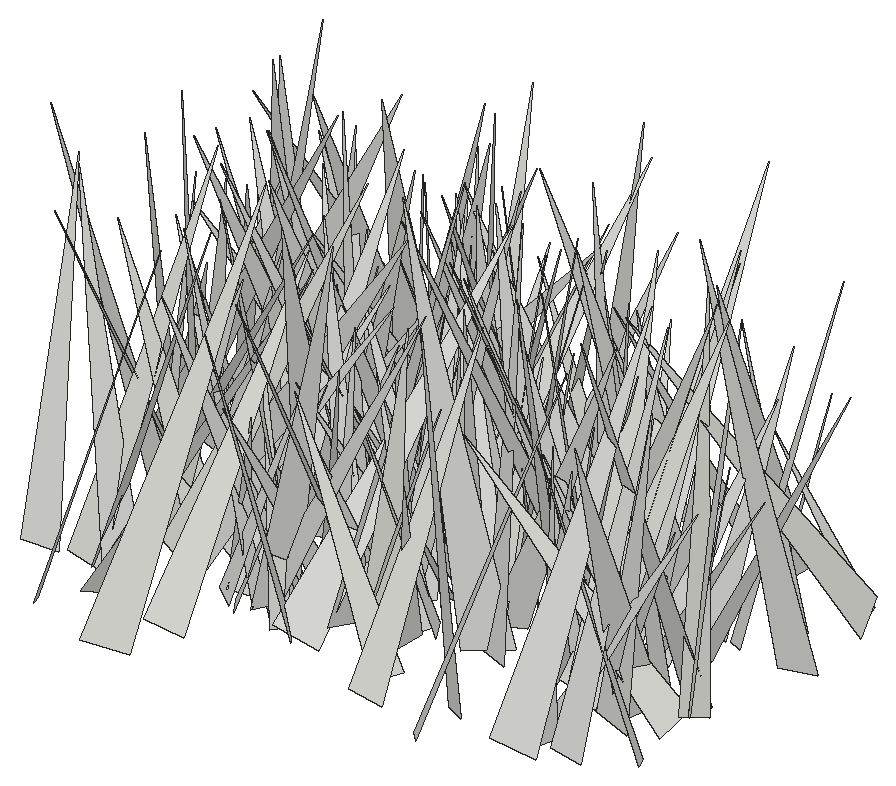
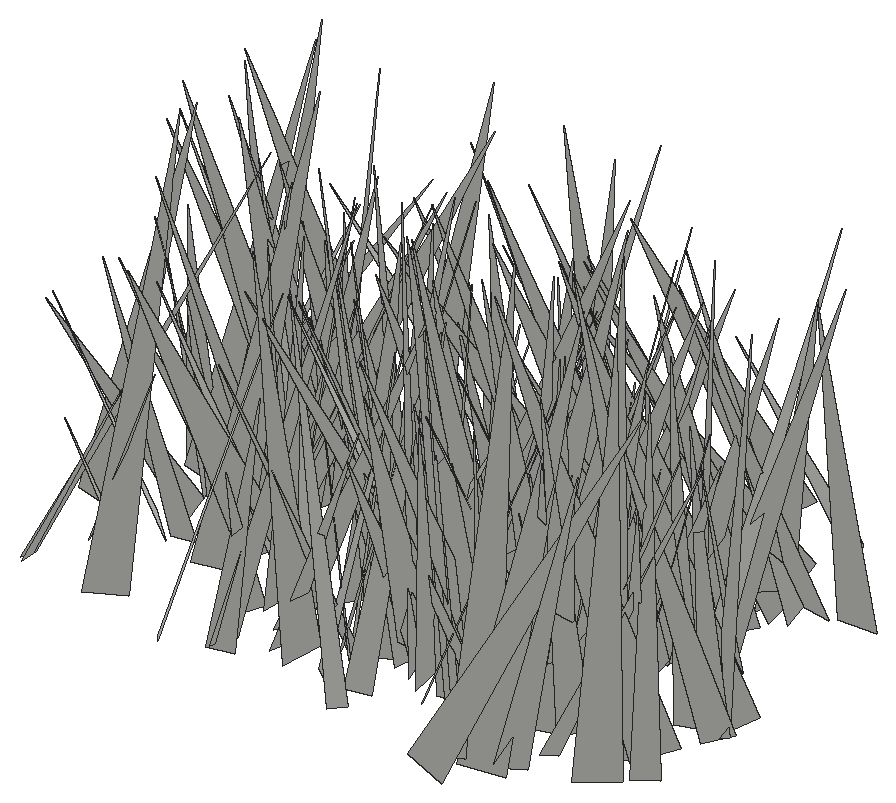
# SketchUp Ruby script. Lengths in inches.
U = 1.inch
M = Sketchup.active_model
def pt(a) = Geom::Point3d.new(a.map { |v| v * U })
def face(e, loops, mat)
  f = e.add_face(loops[0].map { |a| pt(a) })
  loops[1..].each { |l| e.add_face(l.map { |a| pt(a) }).erase! }
  f.material = f.back_material = mat if mat
  f
end
# faces: each face lists its corners as indices into pts; further lists are holes
def faces(e, pts, list, mat = nil) = list.each { |f| face(e, (f[0].is_a?(Array) ? f : [f]).map { |l| l.map { |i| pts[i] } }, mat) }
# xy, xz, yz: faces in a plane at the given z, y or x. An outline is a flat list of corners, or four numbers for a rectangle; further outlines are holes
def ring(l) = l.size == 4 ? [[l[0], l[1]], [l[2], l[1]], [l[2], l[3]], [l[0], l[3]]] : l.each_slice(2).to_a
def flat(e, list, mat, &to3) = list.each { |f| face(e, (f[0].is_a?(Array) ? f : [f]).map { |l| ring(l).map { |u, v| to3.(u, v) } }, mat) }
def xy(e, z, list, mat = nil) = flat(e, list, mat) { |x, y| [x, y, z] }
def xz(e, y, list, mat = nil) = flat(e, list, mat) { |x, z| [x, y, z] }
def yz(e, x, list, mat = nil) = flat(e, list, mat) { |y, z| [x, y, z] }
def lines(e, pts, list) = list.each { |a, b| e.add_line(pt(pts[a]), pt(pts[b])) }
# prism: a flat outline (further loops are holes) pulled along v
def prism(e, loops, v, mat = nil)
  f = face(e, loops, mat); d = Geom::Vector3d.new(v.map { |x| x * U })
  f.pushpull(f.normal.samedirection?(d) ? d.length : -d.length)
end
def box(e, o, s, mat = nil) = prism(e, [[o, [o[0] + s[0], o[1], o[2]], [o[0] + s[0], o[1] + s[1], o[2]], [o[0], o[1] + s[1], o[2]]]], [0, 0, s[2]], mat)
def at(x, y, z, deg = 0) = Geom::Transformation.translation(pt([x, y, z])) * Geom::Transformation.rotation(ORIGIN, Z_AXIS, deg.degrees)
def axes(o, x, y, z) = Geom::Transformation.new([*x, 0, *y, 0, *z, 0, *pt(o).to_a, 1])
def part(name) = M.definitions.add(name)
# library, detail: a bought-in or finely detailed component or shape, given as its bounding box
def library(name, o, s) = part(name).tap { |d| box(d.entities, o, s) }
def detail(e, o, s) = box(e.add_group.entities, o, s)
def put(e, d, t, mat = nil) = e.add_instance(d, t).tap { |i| i.material = mat if mat }
def group(e, t, mat = nil) = e.add_group.tap { |g| g.transformation = t; g.material = mat if mat }.entities
root = M.entities
c1 = part("fur_instance\#9")
p = [[0.8125,0,1.79],[0.67,-0.02,1.48],[0,-0.11,0],[0,0.11,0]]
faces(c1.entities,p,[[0,1,2,3]])
put(root,c1,axes([488.93,113.31,-21.86],[-4.48858,-3.56813,1.07524],[-3.58767,4.5928,0.2643],[1.00813,0.45789,5.72792]))
put(root,c1,axes([485.14,108.57,-21.66],[-5.76444,5.45156,1.05869],[4.71185,5.60881,-3.22628],[2.93919,1.70025,7.24841]))
put(root,c1,axes([481.52,109.58,-21.66],[4.88269,3.53574,0.69101],[3.04894,-4.67553,2.3797],[-1.91908,1.56767,5.53887]))
put(root,c1,axes([493.38,112.67,-21.66],[-3.16425,3.77948,0.90882],[3.82647,2.82214,1.58634],[-0.68447,-1.69527,4.66695]))
put(root,c1,axes([496.26,112.49,-21.86],[-3.8782,-4.63911,2.52217],[-5.26639,3.62608,-1.42825],[0.38461,2.87286,5.87554]))
put(root,c1,axes([489.98,115.99,-21.86],[-3.38776,-6.42257,0.32475],[-6.36234,3.40084,0.88702],[0.93573,-0.12917,7.20691]))
put(root,c1,axes([496.47,110.2,-21.66],[4.76717,4.34009,0.09976],[4.0907,-4.54047,2.05487],[-1.45344,1.45601,6.11063]))
put(root,c1,axes([500.88,116.2,-21.86],[5.9537,-4.05045,0.58701],[-3.75603,-5.81897,-2.05648],[-1.62572,-1.38951,6.90098]))
put(root,c1,axes([485.61,110.99,-21.86],[-1.05391,6.67902,0.37292],[6.52998,1.10912,-1.41007],[1.4518,-0.14015,6.613]))
put(root,c1,axes([492.27,115.18,-21.86],[3.94789,-1.4658,0.35037],[-1.34081,-3.86465,-1.06014],[-0.68816,-0.87925,4.0756]))
put(root,c1,axes([493.44,111.47,-21.86],[0.40052,6.46259,0.29319],[6.45769,-0.38185,-0.40475],[0.38629,-0.31712,6.46233]))
put(root,c1,axes([487.4,114.37,-21.86],[6.75458,-3.1446,1.55563],[-3.25939,-6.87331,0.25842],[-1.29802,0.89549,7.44621]))
put(root,c1,axes([499.78,112.87,-21.86],[-4.70779,-0.34884,1.44292],[-0.70643,4.74641,-1.15738],[1.30563,1.3103,4.57662]))
put(root,c1,axes([481.1,113.37,-21.86],[6.34041,1.92452,0.88463],[1.94009,-6.39712,0.01179],[-0.84995,-0.24555,6.62604]))
put(root,c1,axes([488.49,115.94,-21.66],[1.56687,-4.2825,0.24372],[-4.04586,-1.5617,-1.43053],[-1.42486,-0.27491,4.32996]))
put(root,c1,axes([479.15,112.72,-21.86],[-0.4945,6.57851,1.5324],[6.75453,0.47319,0.14829],[-0.03697,-1.53911,6.5954]))
put(root,c1,axes([502.92,113.63,-21.86],[-4.67684,-2.75,0.36196],[-2.71074,4.38122,-1.73872],[-0.58771,1.67594,5.13928]))
put(root,c1,axes([499.16,111.81,-21.86],[-0.59068,7.87895,1.19707],[7.83923,0.79048,-1.33468],[1.43434,-1.07565,7.78752]))
put(root,c1,axes([482.1,113.25,-21.86],[-6.40273,2.01611,1.14645],[1.98655,6.50456,-0.34415],[1.19695,-0.01086,6.70383]))
put(root,c1,axes([482.37,111.43,-21.86],[6.45135,0.1489,0.38361],[-0.04006,-5.77049,2.9136],[-0.40954,2.91007,5.75787]))
put(root,c1,axes([487.14,114.28,-21.86],[5.1253,5.35023,0.94765],[5.22805,-4.50107,-2.86349],[1.48003,-2.62814,6.83331]))
put(root,c1,axes([486.93,115.4,-21.66],[0.61294,-5.47928,1.38132],[-5.30961,-1.0339,-1.7451],[-1.93355,1.10218,5.22999]))
put(root,c1,axes([485.81,113.8125,-21.86],[2.51167,3.62255,0.80621],[3.69421,-2.34748,-0.96099],[0.35452,-1.20325,4.30208]))
put(root,c1,axes([502.45,115.97,-21.66],[-5.96221,1.49508,0.02596],[1.36332,5.39133,2.61894],[-0.61423,-2.54602,5.56097]))
put(root,c1,axes([499.32,113.95,-21.66],[3.29682,4.04593,0.27696],[3.82738,-2.98619,-1.93627],[1.34069,-1.42422,4.84659]))
put(root,c1,axes([500.63,115.05,-21.86],[1.5633,5.69815,3.01797],[6.40687,-1.02237,-1.38843],[0.72737,-3.24142,5.74326]))
put(root,c1,axes([486.48,113.51,-21.86],[3.52648,2.43175,0.31475],[2.41999,-3.54045,0.23962],[-0.3951,0.0194,4.27692]))
put(root,c1,axes([490.52,114.94,-21.86],[4.57096,2.53062,0.74602],[2.63797,-4.36083,-1.37058],[0.04077,-1.55993,5.04174]))
put(root,c1,axes([484.98,115.65,-21.86],[3.65052,-1.24636,0.3015],[-1.17659,-3.61738,-0.70767],[-0.50984,-0.576,3.79195]))
put(root,c1,axes([488.52,113.33,-21.86],[-4.58917,0.765,0.19448],[0.68534,4.43094,-1.25723],[0.3916,1.21042,4.47941]))
put(root,c1,axes([500.81,112.47,-21.86],[1.7832,7.11152,0.69499],[7.11724,-1.83129,0.47737],[-0.63379,-0.55606,7.31612]))
put(root,c1,axes([480.73,118.375,-21.66],[-3.5223,-6.70382,0.02091],[-6.50166,3.42181,1.83516],[1.63401,-0.83562,7.34711]))
put(root,c1,axes([481.7,113.31,-21.86],[7.04502,0.38941,0.11832],[0.34745,-6.82295,1.76766],[-0.21195,1.75889,6.83077]))
put(root,c1,axes([487,114.3,-21.86],[-6.17227,-0.98801,0.5453],[-1.07692,6.06305,-1.2042],[0.3373,1.27815,6.13375]))
put(root,c1,axes([490.6,116.27,-21.86],[0.67909,-3.62862,0.46379],[-3.53581,-0.77205,-0.86319],[-0.93808,0.2832,3.58928]))
put(root,c1,axes([481.85,115.28,-21.86],[3.48254,-4.50934,1.30252],[-4.66936,-3.1635,1.53235],[0.47726,1.95368,5.48763]))
put(root,c1,axes([490.87,115.37,-21.86],[3.55242,-4.27149,1.91187],[-4.60398,-3.6203,0.46613],[-0.83917,1.77997,5.53606]))
put(root,c1,axes([483.68,115.79,-21.86],[-5.50696,2.25656,1.40845],[2.52369,5.45565,1.12666],[0.84072,-1.59571,5.84374]))
put(root,c1,axes([480.87,112.85,-21.86],[1.55056,7.17303,0.47228],[7.18686,-1.53634,-0.26142],[0.15632,-0.51668,7.33405]))
put(root,c1,axes([488.2,114.85,-21.86],[-6.23091,-2.8217,1.23434],[-3.03851,6.08694,-1.42355],[0.50305,1.81577,6.69027]))
put(root,c1,axes([492.52,116.3,-21.86],[-3.61255,-2.36918,0.54232],[-2.35627,3.65218,0.25916],[0.59592,0.07847,4.31235]))
put(root,c1,axes([494.5625,116.3,-21.86],[2.49125,-7.31611,3.2771],[-7.62751,-3.2193,-1.38865],[-2.46697,2.5655,7.60286]))
put(root,c1,axes([487.44,116.98,-21.66],[4.97524,0.71585,1.07536],[1.04452,-4.74693,-1.67259],[-0.76015,-1.83742,4.74004]))
put(root,c1,axes([489.52,115,-21.86],[1.36793,4.62634,1.5435],[4.80198,-1.5578,0.41343],[-0.85231,-1.35162,4.8066]))
put(root,c1,axes([483.49,115.43,-21.86],[4.41498,5.25807,0.18984],[4.81628,-3.93899,-2.90917],[2.11822,-2.00311,6.21901]))
put(root,c1,axes([483.26,114.58,-21.66],[2.59444,7.48207,1.23534],[7.31718,-2.12705,-2.48457],[1.99156,-1.93206,7.51927]))
put(root,c1,axes([501.62,118.1,-21.86],[-2.16653,-7.31637,0.90738],[-7.36569,2.18851,0.05952],[0.3151,0.85299,7.63018]))
put(root,c1,axes([499.83,115.74,-21.86],[3.74369,-0.67268,0.40161],[-0.71907,-3.7286,0.45768],[-0.31101,0.52348,3.776]))
put(root,c1,axes([496.68,116.57,-21.86],[4.0424,-1.6774,0.68877],[-1.67315,-4.09915,-0.16314],[-0.69903,0.11126,4.37357]))
put(root,c1,axes([481.73,116.35,-21.86],[-2.64388,-6.79077,2.11498],[-6.99476,2.07362,-2.08599],[-1.28885,2.67645,6.98236]))
put(root,c1,axes([492.15,115.99,-21.86],[-4.10178,1.61092,0.95507],[1.70987,4.15942,0.32775],[0.76391,-0.66031,4.39457]))
put(root,c1,axes([496.39,117.84,-21.86],[-6.11732,-3.75265,2.76683],[-3.28898,6.70851,1.82699],[3.3046,-0.26993,6.94018]))
put(root,c1,axes([500.66,117.15,-21.86],[-4.68733,-0.90911,0.30449],[-0.85582,4.65242,0.7161],[0.43216,-0.64711,4.72067]))
put(root,c1,axes([490.16,115.12,-21.66],[-1.21025,6.4146,1.42422],[6.45546,0.89059,1.47445],[-1.22575,-1.64315,6.35907]))
put(root,c1,axes([497.54,116.33,-21.86],[4.4988,1.24272,1.44893],[1.33102,-4.70119,-0.10058],[-1.36826,-0.48722,4.6662]))
put(root,c1,axes([499.07,115.61,-21.86],[0.33091,4.05955,1.18914],[3.81261,-0.80293,1.68011],[-1.83248,-0.93747,3.71034]))
put(root,c1,axes([485.53,119.12,-21.86],[6.57894,-4.30915,0.69378],[-4.10201,-6.53322,-1.6802],[-1.49116,-1.03963,7.68298]))
put(root,c1,axes([490.39,118.65,-21.86],[-4.30266,-2.43803,0.04686],[-2.30354,4.09498,1.544],[0.79994,-1.32144,4.69819]))
put(root,c1,axes([489.26,113.13,-21.86],[-2.37553,7.32496,0.20013],[6.77476,2.27563,-2.87444],[2.79244,0.71043,7.14393]))
put(root,c1,axes([491.4375,118.21,-21.86],[-2.79932,-5.24784,0.26282],[-5.09915,2.64134,-1.57068],[-1.26789,0.96362,5.73663]))
put(root,c1,axes([482.07,117.38,-21.86],[5.30447,3.34271,0.68413],[3.37643,-4.96043,-1.94241],[0.49141,-1.99988,5.96139]))
put(root,c1,axes([490.11,114.375,-21.66],[7.12046,1.58475,2.39098],[0.70942,-7.17277,2.64146],[-2.77938,2.22916,6.79964]))
put(root,c1,axes([497.89,118.59,-21.66],[-2.49506,-7.82927,1.12782],[-7.54738,2.00233,-2.79687],[-2.3678,1.86761,7.7266]))
put(root,c1,axes([482.18,117.92,-21.86],[3.5795,-7.50714,1.0436],[-6.77337,-2.6505,4.166],[3.40115,2.62237,7.19823]))
put(root,c1,axes([490.05,118.02,-21.86],[3.54062,0.10617,1.20258],[0.38468,-3.63127,-0.812],[-1.14433,-0.89222,3.44788]))
put(root,c1,axes([499.27,115.43,-21.86],[6.03648,4.13261,1.07509],[4.02235,-6.12795,0.97074],[-1.43354,0.20766,7.25088]))
put(root,c1,axes([497.41,118.28,-21.86],[4.87258,-2.82126,2.84071],[-2.53321,-5.63755,-1.25383],[-3.10033,0.17232,5.48903]))
put(root,c1,axes([486.5,114.37,-21.86],[-4.73234,6.09922,1.47861],[5.53404,4.92888,-2.61961],[2.95993,0.53615,7.26177]))
put(root,c1,axes([495.06,115.98,-21.86],[2.9733,6.47594,2.08154],[6.51847,-3.36189,1.14821],[-1.94427,-1.36785,7.03277]))
put(root,c1,axes([484.18,115.9,-21.66],[1.81357,5.35205,0.20733],[5.12174,-1.66889,-1.72019],[1.56691,-0.73948,5.38279]))
put(root,c1,axes([499.48,115.35,-21.86],[-5.06165,5.7028,1.49455],[5.55918,5.27278,-1.292],[1.96243,-0.22764,7.51486]))
put(root,c1,axes([498.75,115.8,-21.66],[-0.63507,6.95916,1.46669],[6.78735,1.03289,-1.962],[2.12438,-1.21968,6.70699]))
put(root,c1,axes([494.3,117.6,-21.66],[5.13759,-3.83835,0.8309],[-3.9202,-4.93031,1.46363],[0.23526,1.66651,6.24384]))
put(root,c1,axes([487.75,118.9,-21.86],[-1.12897,-3.54048,0.33773],[-3.515,1.16474,0.46018],[0.54205,0.17891,3.68752]))
put(root,c1,axes([497.3,117.3,-21.86],[6.69732,-3.52244,1.21858],[-3.71872,-6.48437,1.69431],[-0.25228,2.07171,7.37503]))
put(root,c1,axes([498.59,118.43,-21.66],[-4.44374,-5.75342,0.61079],[-5.6055,4.0905,-2.25122],[-1.43294,1.84058,6.91236]))
put(root,c1,axes([497.67,118.74,-21.86],[-6.50715,-2.26194,0.29712],[-2.26712,6.51165,-0.07913],[0.25462,0.17236,6.88863]))
put(root,c1,axes([491.89,119.08,-21.86],[-1.49561,-5.63035,1.67127],[-5.71638,1.79132,0.91926],[1.34798,1.34949,5.75262]))
put(root,c1,axes([494.04,117,-21.86],[-0.34341,4.80516,0.97397],[4.88667,0.41477,-0.32328],[0.39826,-0.94579,4.80656]))
put(root,c1,axes([481.03,118.4375,-21.86],[-4.49865,-5.44108,2.87885],[-5.83326,4.90701,0.15896],[1.96626,2.10876,7.05818]))
put(root,c1,axes([491.21,119.22,-21.86],[-0.33006,-3.76044,0.39687],[-3.50265,0.15395,-1.45434],[-1.42474,0.49269,3.4835]))
put(root,c1,axes([493.96,119.54,-21.66],[-2.04339,-2.88899,0.9747],[-2.5158,2.26047,1.42575],[1.7225,-0.12566,3.23866]))
put(root,c1,axes([489.81,119.75,-21.66],[-2.55131,-7.67351,1.38924],[-7.65133,2.18082,-2.00574],[-1.50657,1.91917,7.83383]))
put(root,c1,axes([497.16,118.72,-21.86],[-5.04486,-3.51647,1.75014],[-3.733,5.17856,-0.35556],[1.22196,1.30239,6.1392]))
put(root,c1,axes([489.57,116.08,-21.86],[-7.91635,-0.39433,1.24518],[-0.80795,7.48837,-2.76517],[1.02625,2.85367,7.42819]))
put(root,c1,axes([487.76,119.1,-21.86],[2.4486,-4.30122,0.69777],[-4.269,-2.2075,1.37318],[0.8735,1.26866,4.75506]))
put(root,c1,axes([500.3,117.96,-21.86],[1.91991,5.69676,2.84026],[5.7974,-2.78995,1.67703],[-2.62873,-1.9923,5.77292]))
put(root,c1,axes([482.73,116.5625,-21.66],[-4.41851,1.16155,1.66424],[0.34777,4.36157,-2.12081],[1.99949,1.8082,4.04655]))
put(root,c1,axes([486.46,117.79,-21.86],[3.13129,2.44329,0.37399],[2.42945,-3.15346,0.26073],[-0.45532,-0.0231,3.96316]))
put(root,c1,axes([489.34,118.85,-21.86],[-3.1283,2.85302,0.75954],[2.94685,2.94951,1.058],[-0.18092,-1.28978,4.09959]))
put(root,c1,axes([500.76,118.85,-21.86],[3.70099,1.78589,1.07617],[1.91017,-3.78303,-0.29128],[-0.83593,-0.7377,4.09901]))
put(root,c1,axes([485.89,118.75,-21.86],[3.11489,-2.67244,0.85057],[-2.80172,-2.90834,1.1224],[0.12545,1.40269,3.94774]))
put(root,c1,axes([480.8,116.8,-21.86],[2.37609,4.94692,0.8109],[4.47755,-2.49789,2.11838],[-2.25414,0.25283,5.06264]))
put(root,c1,axes([482.96,118.42,-21.86],[-2.13288,4.47426,0.69403],[4.36785,1.83113,1.61826],[-1.19274,-1.2953,4.68502]))
put(root,c1,axes([490.71,117.43,-21.86],[-5.11212,3.73872,1.49873],[3.53116,5.32488,-1.23875],[1.93782,0.15985,6.21106]))
put(root,c1,axes([494.42,121.29,-21.66],[6.71484,1.18998,0.43364],[1.2609,-6.06064,-2.89345],[0.11927,-2.92333,6.1752]))
put(root,c1,axes([491.78,117.53,-21.66],[-6.04222,-2.58238,2.07365],[-3.21518,5.60869,-2.38377],[0.79453,3.05796,6.1233]))
put(root,c1,axes([478.36,120.63,-21.86],[-2.86307,-5.78602,1.82095],[-5.78172,3.21211,1.11581],[1.83453,1.09334,6.35847]))
put(root,c1,axes([502.31,116.64,-21.66],[3.51213,5.3509,1.08193],[4.75447,-3.63032,2.52063],[-2.68285,0.57134,5.88334]))
put(root,c1,axes([481.92,120.54,-21.86],[-3.92886,-2.51502,0.86647],[-2.44083,4.02285,0.60923],[1.05758,-0.05874,4.62495]))
put(root,c1,axes([502.63,116.74,-21.66],[-7.06937,0.92542,0.80535],[0.55425,6.6114,-2.73188],[1.09444,2.62944,6.58553]))
put(root,c1,axes([485.24,122.6,-21.86],[6.13444,-4.45258,1.42838],[-3.84619,-6.14459,-2.6359],[-2.65943,-1.38408,7.10696]))
put(root,c1,axes([499.23,118.96,-21.86],[3.6219,-1.04912,0.12415],[-1.02885,-3.40219,1.26523],[0.23987,1.24847,3.55218]))
put(root,c1,axes([490.72,117.21,-21.86],[6.48387,0.57283,2.72889],[-0.5216,-6.53637,2.61139],[-2.73914,2.60063,5.96233]))
put(root,c1,axes([477.86,121.54,-21.66],[0.93957,-4.99379,0.05949],[-4.70596,-0.86502,1.71172],[1.67197,0.37157,4.78443]))
put(root,c1,axes([497.42,122.45,-21.86],[3.52334,-7.25518,1.10129],[-7.15699,-3.66725,-1.26216],[-1.62106,0.42196,7.96608]))
put(root,c1,axes([489.8,119.44,-21.66],[-1.66543,4.2087,0.7623],[4.0491,1.28782,1.73616],[-1.37806,-1.30242,4.18002]))
put(root,c1,axes([485.36,122.12,-21.86],[-6.61379,-2.13915,0.88077],[-1.88588,6.53057,1.69974],[1.33985,-1.36736,6.74011]))
put(root,c1,axes([479.26,121.18,-21.86],[-0.17668,-5.97479,1.5156],[-5.97573,0.53792,1.42395],[1.51188,1.4279,5.80532]))
put(root,c1,axes([484.14,121.95,-21.66],[-0.53016,-5.209,0.61736],[-4.97847,0.69512,1.58982],[1.65216,0.4231,4.98871]))
put(root,c1,axes([483.92,122.5,-21.86],[0.79588,-7.21699,0.96951],[-7.03929,-1.01213,-1.75565],[-1.86367,0.74092,7.04528]))
put(root,c1,axes([478.04,120.32,-21.86],[7.56022,-3.29271,0.03526],[-3.23696,-7.41517,1.59297],[0.60437,1.47429,8.09082]))
put(root,c1,axes([493.12,118.2,-21.86],[-1.83761,6.5724,0.07775],[6.30696,1.74042,1.94227],[-1.85059,-0.59481,6.54223]))
put(root,c1,axes([499.25,119.02,-21.66],[0.30593,5.01742,0.69432],[4.86404,-0.09691,-1.44288],[1.4134,-0.75252,4.8152]))
put(root,c1,axes([486.94,119.67,-21.86],[-3.18645,2.79123,0.05753],[2.78151,3.16651,0.42911],[-0.23972,-0.36053,4.21429]))
put(root,c1,axes([483.65,122.22,-21.66],[5.31663,-1.02418,0.76649],[-0.77202,-5.18142,-1.56841],[-1.02002,-1.41668,5.18224]))
put(root,c1,axes([491.88,121.48,-21.66],[6.71325,2.37054,1.67819],[2.73448,-6.58312,-1.63968],[-0.97898,-2.13225,6.9281]))
put(root,c1,axes([498.29,118.42,-21.86],[1.83288,7.01444,0.75411],[7.05484,-1.82448,-0.17632],[-0.01908,-0.77421,7.24781]))
put(root,c1,axes([482.84,120.81,-21.86],[4.14208,3.82367,0.06036],[3.46383,-3.71363,-2.44781],[1.62049,-1.8356,5.07794]))
put(root,c1,axes([503.125,121.39,-21.86],[-1.04276,-7.37455,2.60053],[-7.71345,0.53914,-1.56404],[-1.28435,2.74945,7.28184]))
put(root,c1,axes([492.52,121.31,-21.86],[-5.43342,3.18473,2.47254],[3.60205,5.6984,0.57576],[1.81141,-1.77869,6.27161]))
put(root,c1,axes([484.79,121.2,-21.86],[6.6153,-1.38256,1.33275],[-1.44359,-6.733,0.18083],[-1.26639,0.45296,6.75581]))
put(root,c1,axes([490.99,124.2,-21.86],[-6.12859,-4.53414,1.24355],[-3.97845,6.08997,2.59781],[2.50535,-1.42065,7.16724]))
put(root,c1,axes([490.59,121.78,-21.86],[5.36268,3.16176,1.79895],[3.56295,-5.21159,-1.4615],[-0.73371,-2.1986,6.05138]))
put(root,c1,axes([482.12,119.375,-21.86],[-7.4216,0.05563,3.73189],[-0.80703,8.0859,-1.72548],[3.64401,1.90407,7.21845]))
put(root,c1,axes([498.29,121.02,-21.86],[4.13039,-0.87619,1.21239],[-0.99071,-4.26996,0.28929],[-1.12075,0.54542,4.21238]))
put(root,c1,axes([495.51,121.36,-21.86],[-3.24328,-4.06122,2.56752],[-4.33534,3.80899,0.54855],[2.07134,1.61325,5.16831]))
put(root,c1,axes([491.21,121.44,-21.86],[-0.52973,-5.32119,2.08202],[-5.65742,0.19488,-0.94137],[-0.8022,2.1395,5.26399]))
put(root,c1,axes([491.87,119.875,-21.86],[4.69636,2.95892,0.9191],[2.85112,-4.78039,0.82137],[-1.21287,0.21986,5.48965]))
put(root,c1,axes([483.36,121.47,-21.86],[-4.7653,3.97573,1.88545],[4.327,4.73874,0.94381],[0.79899,-1.95123,6.13381]))
put(root,c1,axes([477.76,121.52,-21.66],[2.95683,-4.48742,1.40063],[-4.613,-2.45121,1.88504],[0.90496,2.16707,5.03253]))
put(root,c1,axes([487.36,119.07,-21.86],[3.44077,4.42208,0.21812],[4.18127,-3.33634,1.68138],[-1.45578,0.8691,5.34478]))
put(root,c1,axes([485.64,120.25,-21.86],[-4.4668,1.24969,0.75909],[0.98308,4.37301,-1.41442],[1.08236,1.18546,4.4174]))
put(root,c1,axes([486.67,125.41,-21.66],[-5.64756,-4.03637,0.24701],[-3.60758,5.22048,2.82493],[1.82721,-2.16853,6.3409]))
put(root,c1,axes([502.6875,125.54,-21.86],[-7.29463,-2.71144,0.02018],[-2.47986,6.69465,3.09773],[1.09665,-2.89718,7.13916]))
put(root,c1,axes([500.34,120.02,-21.86],[5.03908,0.51167,0.65236],[0.18588,-4.61324,2.18248],[-0.80798,2.12978,4.57066]))
put(root,c1,axes([488.36,121.88,-21.86],[-1.6675,3.7386,1.84502],[3.94069,2.06209,-0.61692],[1.36097,-1.39013,4.04687]))
put(root,c1,axes([490.72,122.02,-21.86],[-3.99392,-3.16377,0.39905],[-3.06383,3.62986,-1.88605],[-0.88412,1.71311,4.73326]))
put(root,c1,axes([483.02,121.98,-21.86],[-5.83458,-0.97839,0.23219],[-1.00024,5.78729,-0.74851],[0.10327,0.77686,5.8685]))
put(root,c1,axes([487.4,121.13,-21.86],[2.13777,3.57515,0.4757],[3.58502,-2.16686,0.17428],[-0.39447,-0.3179,4.1619]))
put(root,c1,axes([489.31,123.55,-21.86],[3.86717,-5.0611,1.49434],[-5.13106,-4.03908,-0.40116],[-1.23289,0.93486,6.35679]))
put(root,c1,axes([486.1,121.875,-21.86],[7.6269,-0.50277,1.8471],[-0.68475,-7.80192,0.70374],[-1.78765,0.84341,7.61099]))
put(root,c1,axes([483.05,124.37,-21.86],[4.14575,-5.15062,1.64406],[-4.88287,-4.45639,-1.64839],[-2.32151,0.17524,6.40304]))
put(root,c1,axes([479.85,124.625,-21.86],[7.83218,-2.47016,1.5817],[-2.12062,-7.88445,-1.81244],[-2.02643,-1.29626,8.00998]))
put(root,c1,axes([488.67,126.26,-21.66],[-2.64275,-7.72517,0.10148],[-7.35563,2.5487,2.46402],[2.36287,-0.70608,7.78402]))
put(root,c1,axes([488.92,123.52,-21.86],[6.48852,0.93317,0.66882],[1.0636,-6.33108,-1.48501],[-0.43231,-1.57025,6.38486]))
put(root,c1,axes([499.43,121.67,-21.86],[0.7475,5.23214,1.319],[5.34274,-0.53135,-0.92008],[0.75507,-1.41992,5.20456]))
put(root,c1,axes([488.4375,120.94,-21.86],[-5.56085,2.56326,1.5764],[2.25423,5.74256,-1.38556],[1.99343,0.65656,5.96435]))
put(root,c1,axes([481.52,121.26,-21.86],[-0.14147,5.00237,0.6936],[4.87308,-0.04695,1.33257],[-1.32587,-0.70632,4.82369]))
put(root,c1,axes([488.64,121.53,-21.86],[5.74165,3.30721,0.02247],[3.30582,-5.73764,-0.2359],[0.09829,-0.21562,6.62182]))
put(root,c1,axes([477.97,125,-21.66],[0.06322,-6.05576,0.15688],[-5.74231,-0.00994,1.93043],[1.92942,0.16885,5.74018]))
put(root,c1,axes([496.73,120.49,-21.66],[5.00084,3.55671,0.83126],[3.26277,-4.98345,1.69387],[-1.6418,0.92989,5.89825]))
put(root,c1,axes([488.39,123.6875,-21.86],[7.03768,2.72348,2.80411],[3.28727,-7.24831,-1.21043],[-2.11523,-2.20318,7.44856]))
put(root,c1,axes([499.17,126,-21.86],[6.98894,-3.62557,1.01436],[-3.15649,-6.80873,-2.58782],[-2.05189,-1.87497,7.43594]))
put(root,c1,axes([481.58,125.37,-21.86],[-5.28354,-0.86585,0.73138],[-0.45173,4.80676,2.42722],[1.0395,-2.31209,4.77222]))
put(root,c1,axes([494.51,122.93,-21.86],[-6.58404,0.20466,2.39247],[0.20033,7.00521,-0.04793],[2.39284,-0.02336,6.58705]))
put(root,c1,axes([485.52,124.36,-21.86],[6.15872,-4.73604,0.69713],[-4.78091,-6.14284,0.50431],[-0.2428,0.82545,7.75278]))
put(root,c1,axes([478.7,123.57,-21.66],[4.47531,-6.51665,1.20055],[-6.35255,-3.80729,3.0143],[1.88498,2.64087,7.30815]))
put(root,c1,axes([492.91,124.35,-21.66],[-6.35837,1.48,1.02188],[1.69793,6.17763,1.61781],[0.593,-1.81932,6.3247]))
put(root,c1,axes([485.02,121.48,-21.86],[0.07199,5.81915,0.58708],[5.58747,-0.24194,1.7129],[-1.72841,-0.53974,5.5618]))
put(root,c1,axes([482.69,123.25,-21.86],[2.6007,2.51832,0.88377],[2.64819,-2.58836,-0.41733],[-0.33183,-0.9193,3.59603]))
put(root,c1,axes([489.7,120.78,-21.66],[0.36828,7.38641,0.21711],[7.15433,-0.30198,-1.86176],[1.84979,-0.30261,7.15741]))
put(root,c1,axes([486.15,124.82,-21.66],[-1.36067,-5.7583,1.83351],[-5.61411,1.9,1.80082],[2.23642,1.26617,5.63617]))
put(root,c1,axes([486.64,122.49,-21.86],[-4.83197,-1.5354,1.95575],[-2.0901,4.8234,-1.3772],[1.34681,1.9768,4.87942]))
put(root,c1,axes([494.27,126.08,-21.86],[-7.41474,-1.37074,2.09218],[-0.74138,7.45582,2.25736],[2.38883,-1.94072,7.19456]))
put(root,c1,axes([490.25,124.71,-21.66],[3.23905,1.92957,1.10614],[2.22288,-2.8741,-1.49551],[-0.07469,-1.85863,3.46094]))
put(root,c1,axes([481.84,123.77,-21.86],[5.47744,-1.647,1.93505],[-1.81976,-5.75174,0.25556],[-1.77356,0.81501,5.71398]))
put(root,c1,axes([483.2,122.99,-21.86],[-3.95377,2.90545,0.68572],[2.92437,3.99824,-0.07937],[0.59996,-0.34142,4.90588]))
put(root,c1,axes([490.51,125.8125,-21.86],[-3.60567,-4.25836,0.82426],[-4.10665,3.69659,1.13335],[1.39586,-0.12438,5.46351]))
put(root,c1,axes([490.77,123.91,-21.86],[3.89411,3.28531,3.07479],[3.51498,-4.75969,0.63397],[-2.80935,-1.40135,5.05524]))
put(root,c1,axes([479.29,125.76,-21.86],[5.45655,-4.97036,1.37233],[-4.9464,-5.60993,-0.6508],[-1.45634,0.43117,7.35221]))
put(root,c1,axes([500.52,121.45,-21.86],[3.77258,4.9169,0.38845],[4.64704,-3.70729,1.79444],[-1.65279,0.7995,5.93196]))
put(root,c1,axes([483.9,125.33,-21.66],[5.26826,5.58359,0.80335],[4.69893,-3.73546,-4.8521],[3.1212,-3.80083,5.9488]))
put(root,c1,axes([485.46,123.12,-21.86],[6.3266,0.04535,0.7535],[-0.10627,-6.24313,1.26797],[-0.74735,1.27161,6.1984]))
put(root,c1,axes([496.84,120.69,-21.86],[-5.35866,5.61511,0.59327],[5.12673,5.1813,-2.73266],[2.36603,1.4904,7.2648]))
put(root,c1,axes([483.08,127.36,-21.66],[6.31463,-5.10403,0.36931],[-4.97216,-6.25818,-1.47472],[-1.21044,-0.91981,7.98441]))
put(root,c1,axes([501.91,123.05,-21.66],[-5.07583,-0.99149,0.0646],[-0.93064,4.62637,-2.11704],[-0.34804,2.08923,4.7186]))
put(root,c1,axes([482.65,127.49,-21.86],[1.9178,-7.47283,0.23219],[-7.45531,-1.92947,-0.52008],[-0.56157,0.09505,7.69744]))
put(root,c1,axes([488.62,122.85,-21.86],[-2.91269,3.59929,0.76549],[3.33369,2.99435,-1.39463],[1.55801,0.3218,4.41516]))
put(root,c1,axes([495.84,127.48,-21.66],[-4.51609,-3.87484,0.43498],[-3.47065,4.29803,2.25393],[1.77713,-1.453,5.5072]))
put(root,c1,axes([502.58,125.7,-21.86],[-3.53813,-0.73541,0.01575],[-0.72603,3.50386,0.50526],[0.11809,-0.49152,3.57826]))
put(root,c1,axes([488.79,127.16,-21.86],[6.70588,0.95076,0.50826],[1.07552,-6.12086,-2.74035],[-0.07444,-2.78609,6.19381]))
put(root,c1,axes([492.67,125.12,-21.86],[-4.67838,0.58429,0.4377],[0.60816,4.68963,0.24018],[0.40387,-0.29353,4.7086]))
put(root,c1,axes([487.66,123.96,-21.86],[-5.53054,0.45224,1.5037],[0.10523,5.59989,-1.29715],[1.5667,1.22031,5.39525]))
put(root,c1,axes([500.21,123.68,-21.86],[2.52886,2.74781,0.4271],[2.47453,-2.48701,1.34889],[-1.2687,0.62635,3.48225]))
put(root,c1,axes([490.42,124.16,-21.86],[2.55836,5.15566,0.46861],[5.11042,-2.43162,-1.14739],[0.82709,-0.92305,5.63999]))
put(root,c1,axes([494.85,123.9,-21.86],[-3.06168,2.49465,0.02952],[2.42804,2.99025,-0.87237],[0.57338,0.65813,3.85176]))
put(root,c1,axes([489.08,122.52,-21.86],[-6.53703,2.92768,0.70077],[2.53956,6.26275,-2.47462],[1.61648,2.00045,6.72163]))
put(root,c1,axes([491.77,125.24,-21.86],[6.98669,-0.82296,2.45735],[-1.02769,-7.36659,0.45485],[-2.37901,0.76535,7.02027]))
put(root,c1,axes([493.99,126.6,-21.86],[1.41164,-4.04262,0.99191],[-4.10193,-1.52908,-0.39425],[-0.70768,0.79907,4.26381]))
put(root,c1,axes([484.125,128.52,-21.86],[-0.45254,-7.13046,0.09555],[-6.72101,0.39447,-2.39372],[-2.38342,0.24148,6.7319]))
put(root,c1,axes([482,126.84,-21.86],[3.58153,-3.37168,2.12142],[-3.21603,-4.13077,-1.13573],[-2.3507,0.51427,4.78599]))
